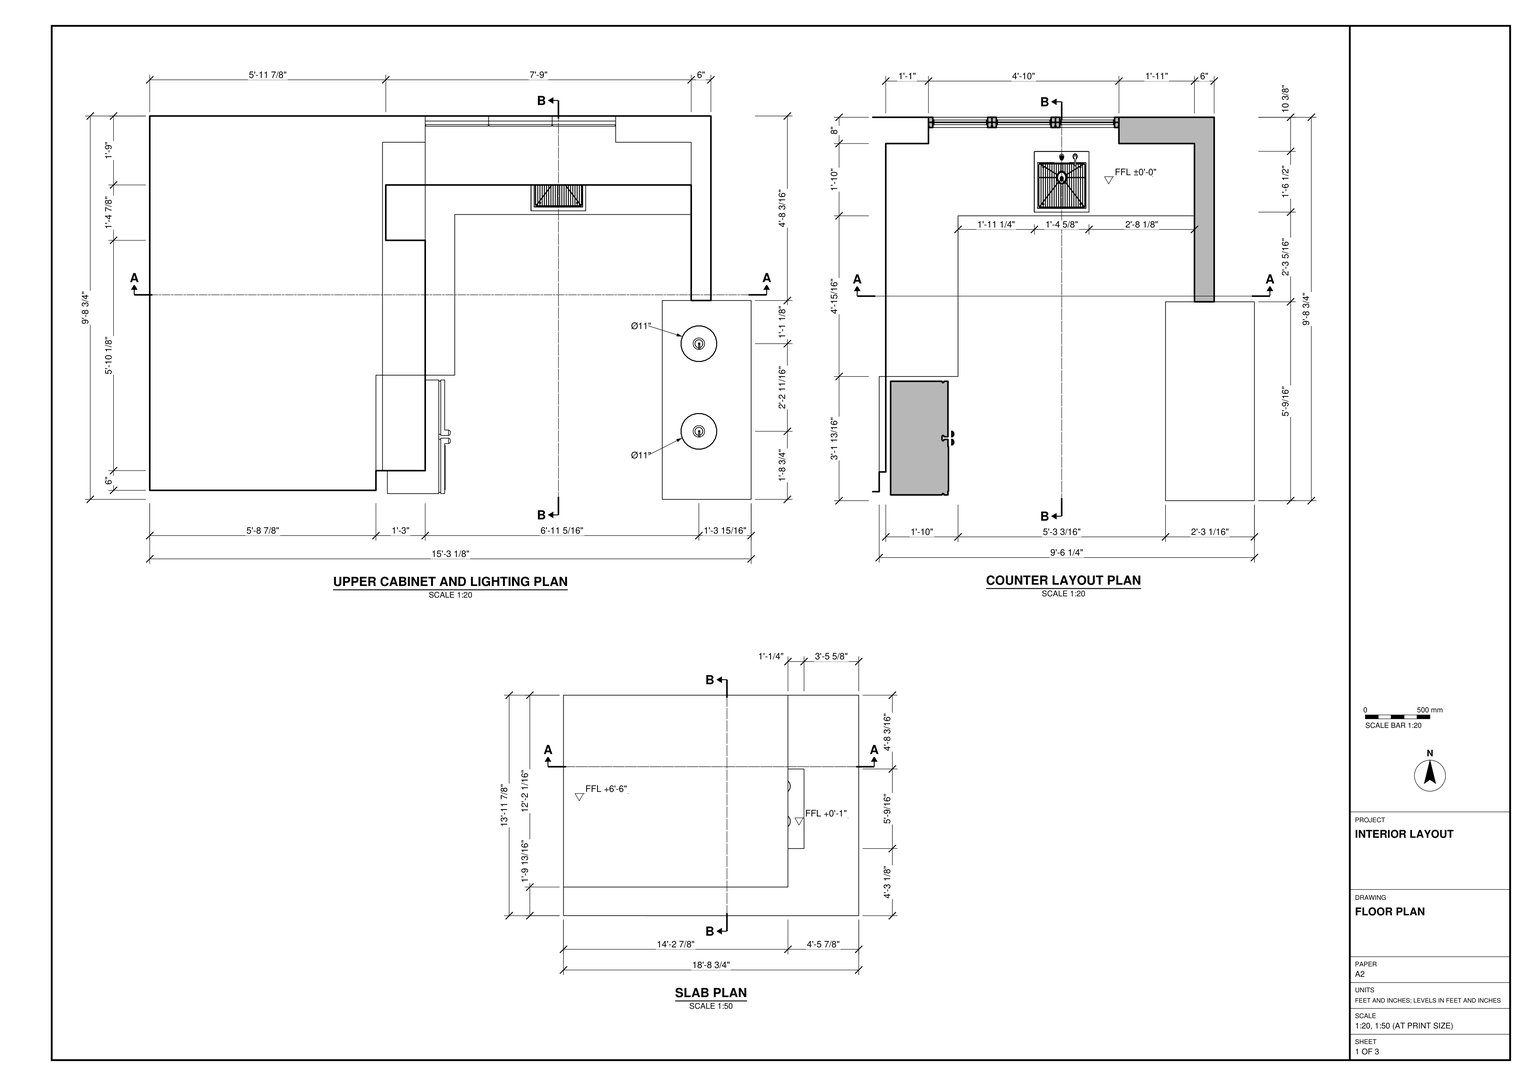
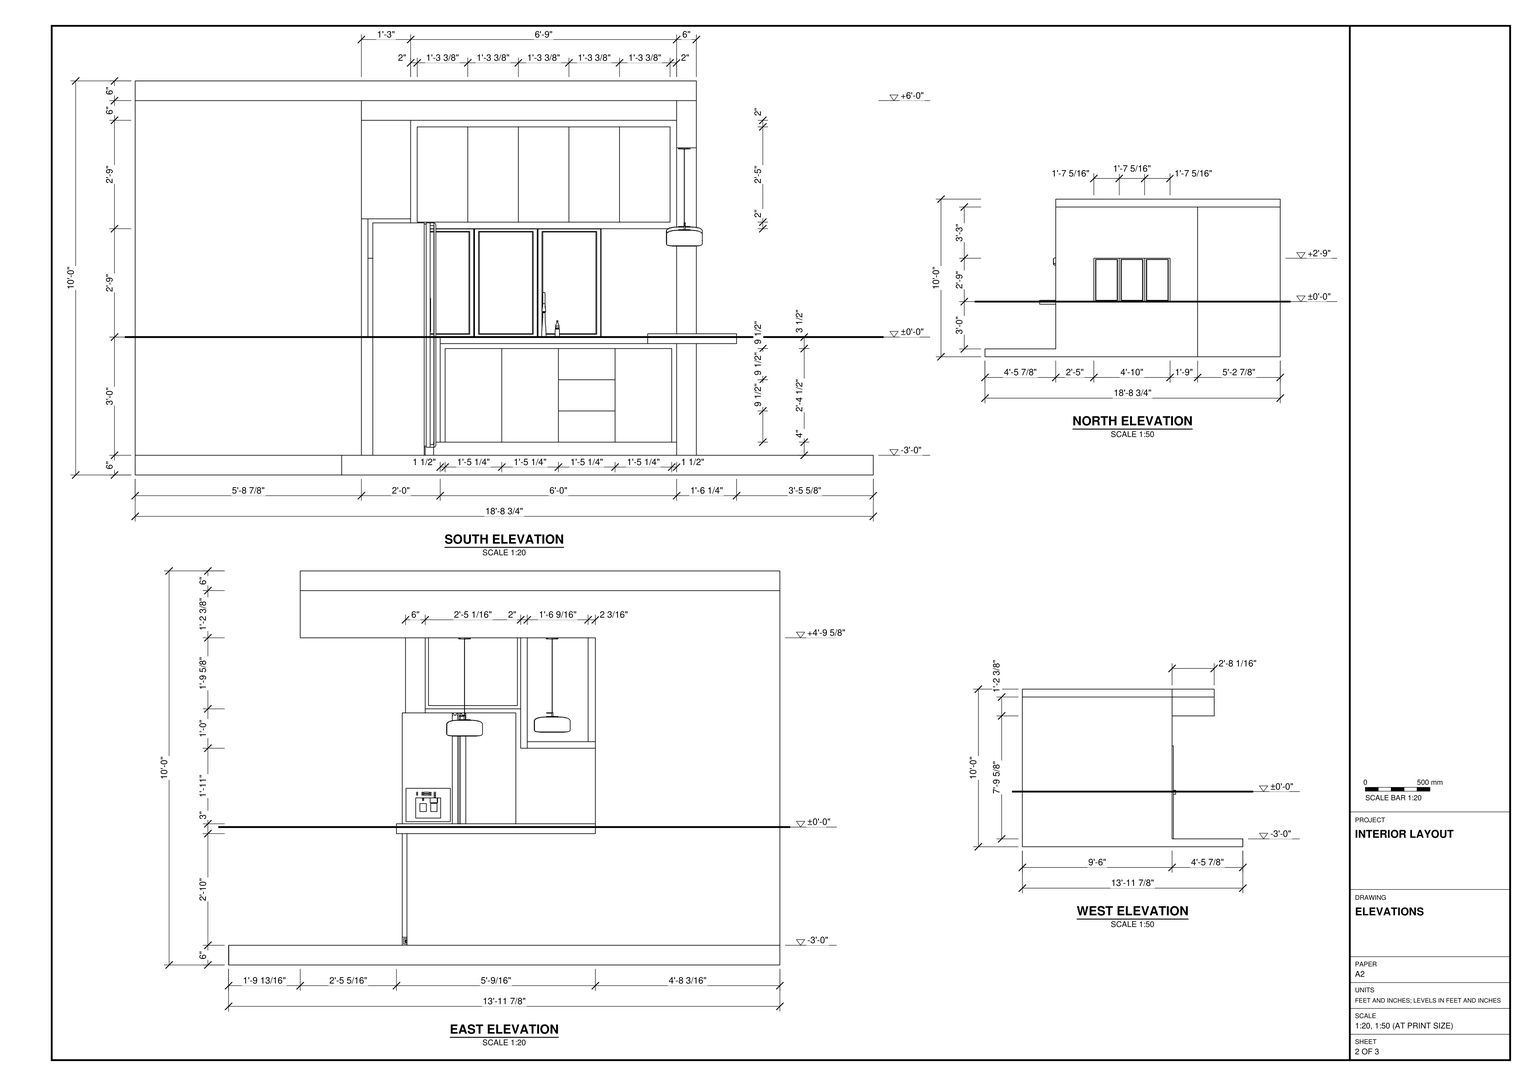
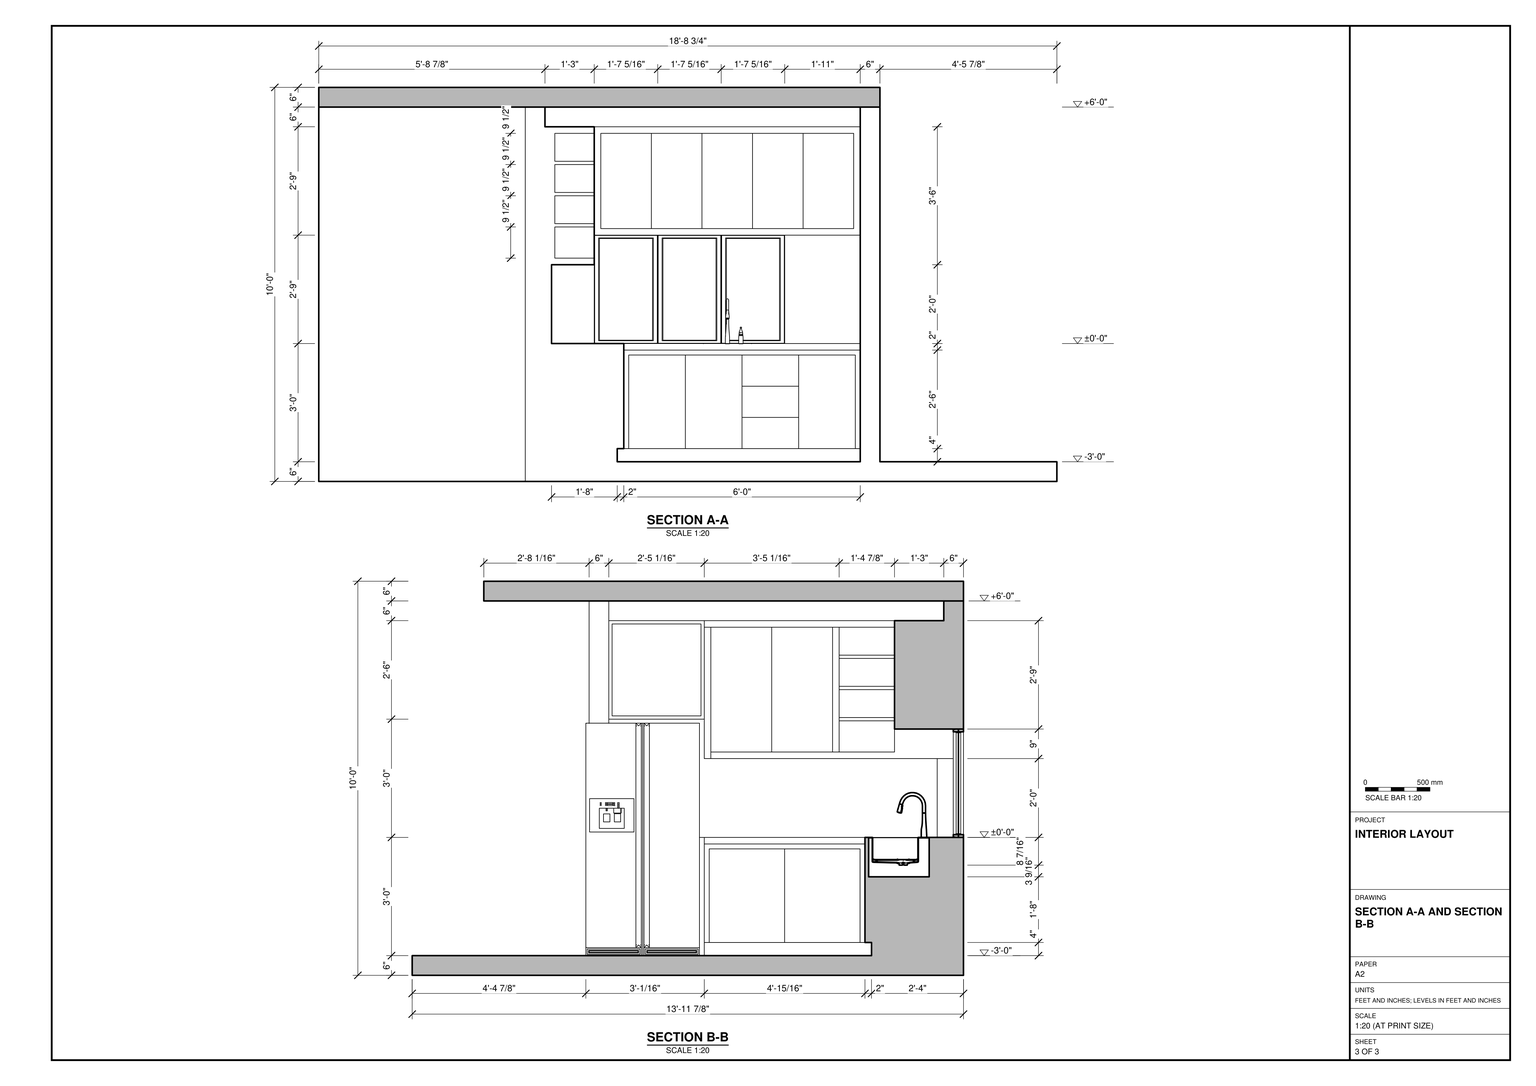
Build the kitchen interior in SketchUp from task_files/diagram_01.pdf. Work in feet and inches. The overall model is 18'-8 3/4" along X, 13'-11 7/8" along Y and 10'-0" high. Use the single reference level ±0'-0" at the sink worktop. The top of the floor slab is at -3'-0" and the underside of the overhead slab is at +6'-0". Use the slab plan for their different footprints and the sections for their thicknesses. Model the walls and returns to the thicknesses drawn, leaving the kitchen open where shown.

Build the L-shaped counter with the sink and faucet below the three-panel window. Follow the elevations for the cupboard fronts, drawer stack and recessed plinth beneath the sink run. Fit the upper cabinets and open shelves around the corner, with space for the tall refrigerator at the end of the return. Place the projecting counter on the opposite side of the aisle and use the lighting plan to position the two lights above it. Appliances, lights, decor and loose items may be any suitable library components.

Keep the walls, floor slab, overhead slab and each furniture or joinery piece in separate groups or components. Use components for repeated parts such as matching cabinet fronts. Save one SketchUp model as output_files/kitchen_with_fitted_cabinets_and_projecting_counter.skp.

# SketchUp Ruby script. Lengths in inches.
U = 1.inch
M = Sketchup.active_model
def pt(a) = Geom::Point3d.new(a.map { |v| v * U })
def face(e, loops, mat)
  f = e.add_face(loops[0].map { |a| pt(a) })
  loops[1..].each { |l| e.add_face(l.map { |a| pt(a) }).erase! }
  f.material = f.back_material = mat if mat
  f
end
# faces: each face lists its corners as indices into pts; further lists are holes
def faces(e, pts, list, mat = nil) = list.each { |f| face(e, (f[0].is_a?(Array) ? f : [f]).map { |l| l.map { |i| pts[i] } }, mat) }
# xy, xz, yz: faces in a plane at the given z, y or x. An outline is a flat list of corners, or four numbers for a rectangle; further outlines are holes
def ring(l) = l.size == 4 ? [[l[0], l[1]], [l[2], l[1]], [l[2], l[3]], [l[0], l[3]]] : l.each_slice(2).to_a
def flat(e, list, mat, &to3) = list.each { |f| face(e, (f[0].is_a?(Array) ? f : [f]).map { |l| ring(l).map { |u, v| to3.(u, v) } }, mat) }
def xy(e, z, list, mat = nil) = flat(e, list, mat) { |x, y| [x, y, z] }
def xz(e, y, list, mat = nil) = flat(e, list, mat) { |x, z| [x, y, z] }
def yz(e, x, list, mat = nil) = flat(e, list, mat) { |y, z| [x, y, z] }
def lines(e, pts, list) = list.each { |a, b| e.add_line(pt(pts[a]), pt(pts[b])) }
# prism: a flat outline (further loops are holes) pulled along v
def prism(e, loops, v, mat = nil)
  f = face(e, loops, mat); d = Geom::Vector3d.new(v.map { |x| x * U })
  f.pushpull(f.normal.samedirection?(d) ? d.length : -d.length)
end
def box(e, o, s, mat = nil) = prism(e, [[o, [o[0] + s[0], o[1], o[2]], [o[0] + s[0], o[1] + s[1], o[2]], [o[0], o[1] + s[1], o[2]]]], [0, 0, s[2]], mat)
def at(x, y, z, deg = 0) = Geom::Transformation.translation(pt([x, y, z])) * Geom::Transformation.rotation(ORIGIN, Z_AXIS, deg.degrees)
def axes(o, x, y, z) = Geom::Transformation.new([*x, 0, *y, 0, *z, 0, *pt(o).to_a, 1])
def part(name) = M.definitions.add(name)
# library, detail: a bought-in or finely detailed component or shape, given as its bounding box
def library(name, o, s) = part(name).tap { |d| box(d.entities, o, s) }
def detail(e, o, s) = box(e.add_group.entities, o, s)
def put(e, d, t, mat = nil) = e.add_instance(d, t).tap { |i| i.material = mat if mat }
def group(e, t, mat = nil) = e.add_group.tap { |g| g.transformation = t; g.material = mat if mat }.entities
root = M.entities
M.materials.add("Wine2").color = [0, 0, 0]
M.materials["Wine2"].alpha = 0
M.materials.add("[0046_Gold]").color = [255, 215, 0]
M.materials.add("[0067_PaleGreen]").color = [152, 251, 152]
M.materials.add("[0070_SpringGreen]").color = [0, 255, 127]
M.materials.add("[0072_DarkSeaGreen]").color = [143, 188, 143]
M.materials.add("[0087_Cyan]").color = [0, 255, 255]
M.materials.add("[0088_Aquamarine]").color = [127, 255, 212]
M.materials.add("[0096_SkyBlue]").color = [135, 206, 235]
M.materials.add("[0117_GhostWhite]").color = [248, 248, 255]
M.materials.add("[0128_White]").color = [255, 255, 255]
M.materials.add("[0130_Gainsboro]").color = [39, 45, 50]
M.materials.add("[0131_Silver]").color = [192, 192, 192]
M.materials.add("[0133_Gray]").color = [128, 128, 128]
M.materials.add("[0134_DimGray]").color = [105, 105, 105]
M.materials.add("[0136_Charcoal]").color = [35, 35, 35]
M.materials.add("[0137_Black]").color = [0, 0, 0]
M.materials.add("[Granite Dark Gray]").color = [69, 68, 68]
c1 = part("Framed glass panel")
xy(c1.entities,0,[[0,-0.98,43.07,0],[0,0,43.07,1.4]],"[0130_Gainsboro]")
xy(c1.entities,0.3,[[0.3,-1.43,42.77,-0.98]],"[0130_Gainsboro]")
xy(c1.entities,2.95,[[2.95,-1.43,40.12,-0.63],[2.95,-0.63,40.12,0],[2.95,0,40.12,0.64],[2.95,0.64,40.12,1.4]],"[0130_Gainsboro]")
xy(c1.entities,3.54,[[3.54,-0.63,39.53,0],[3.54,0,39.53,0.64]],"[0130_Gainsboro]")
xy(c1.entities,111.8125,[[3.54,-0.63,39.53,0],[3.54,0,39.53,0.64]],"[0130_Gainsboro]")
xy(c1.entities,112.4,[[2.95,-1.43,40.12,-0.63],[2.95,-0.63,40.12,0],[2.95,0,40.12,0.64],[2.95,0.64,40.12,1.4]],"[0130_Gainsboro]")
xy(c1.entities,115.05,[[0.3,-1.43,42.77,-0.98]],"[0130_Gainsboro]")
xy(c1.entities,115.35,[[0,-0.98,43.07,0],[0,0,43.07,1.4]],"[0130_Gainsboro]")
xz(c1.entities,-1.43,[[[0.3,0.3,42.77,115.05],[2.95,2.95,40.12,112.4]]],"[0130_Gainsboro]")
xz(c1.entities,-0.98,[[[0,0,43.07,115.35],[0.3,0.3,42.77,115.05]]],"[0130_Gainsboro]")
xz(c1.entities,-0.63,[[[2.95,2.95,40.12,112.4],[3.54,3.54,39.53,111.8125]]],"[0130_Gainsboro]")
xz(c1.entities,0,[[3.54,3.54,39.53,111.8125]],"Wine2")
xz(c1.entities,0,[[[0,0,43.07,115.35],[2.95,2.95,40.12,112.4]],[[2.95,2.95,40.12,112.4],[3.54,3.54,39.53,111.8125]]],"[0130_Gainsboro]")
xz(c1.entities,0.64,[[[2.95,2.95,40.12,112.4],[3.54,3.54,39.53,111.8125]]],"[0130_Gainsboro]")
xz(c1.entities,1.4,[[[0,0,43.07,115.35],[2.95,2.95,40.12,112.4]]],"[0130_Gainsboro]")
yz(c1.entities,0,[[-0.98,0,0,115.35],[0,0,1.4,115.35]],"[0130_Gainsboro]")
yz(c1.entities,0.3,[[-1.43,0.3,-0.98,115.05]],"[0130_Gainsboro]")
yz(c1.entities,2.95,[[-1.43,2.95,-0.63,112.4],[-0.63,2.95,0,112.4],[0,2.95,0.64,112.4],[0.64,2.95,1.4,112.4]],"[0130_Gainsboro]")
yz(c1.entities,3.54,[[-0.63,3.54,0,111.8125],[0,3.54,0.64,111.8125]],"[0130_Gainsboro]")
yz(c1.entities,39.53,[[-0.63,3.54,0,111.8125],[0,3.54,0.64,111.8125]],"[0130_Gainsboro]")
yz(c1.entities,40.12,[[-1.43,2.95,-0.63,112.4],[-0.63,2.95,0,112.4],[0,2.95,0.64,112.4],[0.64,2.95,1.4,112.4]],"[0130_Gainsboro]")
yz(c1.entities,42.77,[[-1.43,0.3,-0.98,115.05]],"[0130_Gainsboro]")
yz(c1.entities,43.07,[[-0.98,0,0,115.35],[0,0,1.4,115.35]],"[0130_Gainsboro]")
c2 = library("3822-1\#1",[-12.47,-11.03,-4.97],[24.94,22.06,9.94])
c3 = library("647\#1",[-5.42,-7.01,-8.07],[10.84,8.15,16.14])
c4 = library("Cubed Ice",[0.01,0,0],[0.63,0.13,0.01])
c5 = library("Crushed Ice",[0.01,0,0],[0.77,0.13,0.01])
c6 = library("Up",[0.01,0,0],[0.17,0.15,0.01])
c7 = library("Down",[0.01,0,0],[0.36,0.12,0.01])
c8 = library("Down\#1",[0.01,0,0],[0.36,0.12,0.01])
c9 = library("Up\#1",[0.01,0,0],[0.17,0.15,0.01])
c10 = library("Temp: 37*",[0.02,0,0],[1.12,0.22,0.01])
c11 = library("Temp: 0*",[0.02,0,0],[0.98,0.22,0.01])
c12 = library("Hold Temperature",[0.01,0,0],[1.21,0.16,0.01])
c13 = library("Deep Freeze",[0.01,0,0],[0.81,0.15,0.01])
c14 = library("Light",[0.01,0,0],[0.32,0.16,0.01])
c15 = library("建立群組\#482",[0,0,0],[10.95,10.95,81.29])
xy(root,0,[[62.875,0,62.875,0.0625,0,0.0625,0,59.875,62.875,59.875,62.875,167.875,224.75,167.875,224.75,0],[0,59.875,62.875,167.875]],"[0128_White]")
xy(root,6,[[[62.875,0,62.875,0.0625,0,0.0625,0,53.875,68.875,53.875,68.875,88.95,90.875,88.95,90.875,139.875,164.875,139.875,164.875,54.3125,170.875,54.3125,170.875,167.875,224.75,167.875,224.75,0],[72.35,52.88,88.31,52.88,88.31,69.77,88,69.77,88,70.59,88.31,70.59,88.31,87.48,72.35,87.48]],[72.35,52.88,72.35,87.48,88.31,87.48,88.31,70.59,88,70.59,88,69.77,88.31,69.77,88.31,52.88]],"[0128_White]")
xy(root,6.41,[[88.01,53.3,88.31,69.36],[88,71.01,88.31,87.07]],"[0137_Black]")
xy(root,6.8125,[[88.01,53.71,88.31,68.95],[88,71.42,88.31,86.66]],"[0137_Black]")
xy(root,7.02,[[88.01,53.91,88.31,68.74],[88,71.625,88.31,86.45]],"[0137_Black]")
xy(root,7.42,[[88.01,53.91,88.31,68.74],[88,71.625,88.31,86.45]],"[0137_Black]")
xy(root,7.62,[[88.01,53.71,88.31,68.95],[88,71.42,88.31,86.66]],"[0137_Black]")
xy(root,8.03,[[88.01,53.3,88.31,69.36],[88,71.01,88.31,87.07]],"[0137_Black]")
xy(root,8.4375,[[88.61,52.88,88.61,69.77,90.95,69.77,90.95,68.12,89.8125,68.12,89.8125,52.88],[88.61,70.59,88.61,87.48,89.8125,87.48,89.8125,72.24,90.95,72.24,90.95,70.59]])
xy(root,8.4375,[[88.01,52.88,88.31,69.77],[88,70.59,88.31,87.48]],"[0137_Black]")
xy(root,9.25,[[89.8125,68.12,91.01,69.77],[89.8125,70.59,91.01,72.24]])
xy(root,10,[[90.875,88.95,92.875,139.875],[92.875,137.875,164.875,139.875]],"[0128_White]")
xy(root,30,[[116.07,138.99,132.75,157.43]],"[0137_Black]")
xy(root,40,[[156.0625,51.125,164.875,111.6875],[164.875,51.125,170.875,54.3125],[170.875,51.125,183.125,111.6875]],"[0137_Black]")
xy(root,42,[[68.875,59.875,70.875,88.95]],"[0128_White]")
xy(root,42,[[[70.875,88.95,92.875,88.95,92.875,137.875,164.875,137.875,164.875,159.875,141.875,159.875,141.875,167.875,83.875,167.875,83.875,159.875,70.875,159.875],[116.07,138.99,132.75,157.43]]],"[0137_Black]")
xy(root,43,[[156.0625,51.125,183.125,111.6875]],"[0137_Black]")
xy(root,43.64,[[89.8125,54.03,89.96,67.54]])
xy(root,44.73,[[88,56.98,89.96,64.58]],"[0136_Charcoal]")
xy(root,46.72,[[88,58.26,88.31,60.22],[88,61.56,88.31,63.48]],"[0134_DimGray]")
xy(root,49.15,[[88,58.26,88.31,60.22]],"[0134_DimGray]")
xy(root,49.21,[[88,61.56,88.31,63.48]],"[0131_Silver]")
xy(root,49.41,[[[88.9375,61.375,88.72,61.43,88.53,61.55,88.36,61.74,88.24,61.99,88.16,62.26,88.14,62.56,88.18,62.85,88.27,63.12,88.41,63.35,88.59,63.52,88.79,63.62,89.01,63.65,89.22,63.6,89.42,63.47,89.59,63.28,89.71,63.04,89.79,62.76,89.8,62.46,89.77,62.17,89.68,61.9,89.54,61.67,89.36,61.5,89.15,61.4],[88.94,61.51,89.13,61.53,89.3125,61.62,89.47,61.77,89.59,61.97,89.67,62.21,89.71,62.47,89.69,62.73,89.625,62.98,89.52,63.19,89.37,63.36,89.19,63.47,89.01,63.52,88.8125,63.49,88.63,63.4,88.48,63.25,88.35,63.05,88.27,62.8125,88.24,62.55,88.26,62.29,88.32,62.05,88.43,61.83,88.58,61.66,88.75,61.55]]])
xy(root,50.09,[[[88.67,59.02,88.64,59.03,88.6,59.05,88.57,59.08,88.54,59.12,88.52,59.22,88.53,59.28,88.54,59.33,88.57,59.37,88.6,59.4,88.64,59.42,88.67,59.43,88.71,59.42,88.75,59.4,88.78,59.37,88.8,59.33,88.82,59.28,88.82,59.17,88.8,59.12,88.78,59.08,88.75,59.05,88.71,59.03],[88.67,59.08,88.73,59.1,88.75,59.125,88.76,59.15,88.77,59.1875,88.78,59.22,88.76,59.3,88.75,59.32,88.73,59.35,88.67,59.37,88.65,59.36,88.62,59.35,88.6,59.32,88.58,59.3,88.57,59.26,88.57,59.1875,88.58,59.15,88.62,59.1,88.65,59.09]]])
xy(root,50.89,[[88.67,59.08,88.65,59.09,88.62,59.1,88.58,59.15,88.57,59.1875,88.57,59.26,88.58,59.3,88.6,59.32,88.62,59.35,88.65,59.36,88.67,59.37,88.73,59.35,88.75,59.32,88.76,59.3,88.78,59.22,88.77,59.1875,88.76,59.15,88.75,59.125,88.73,59.1],[88.94,61.51,88.75,61.55,88.58,61.66,88.43,61.83,88.32,62.05,88.26,62.29,88.24,62.55,88.27,62.8125,88.35,63.05,88.48,63.25,88.63,63.4,88.8125,63.49,89.01,63.52,89.19,63.47,89.37,63.36,89.52,63.19,89.625,62.98,89.69,62.73,89.71,62.47,89.67,62.21,89.59,61.97,89.47,61.77,89.3125,61.62,89.13,61.53]])
xy(root,50.89,[[[88,56.98,89.96,64.58],[88.9375,61.375,89.15,61.4,89.36,61.5,89.54,61.67,89.68,61.9,89.77,62.17,89.8,62.46,89.79,62.76,89.71,63.04,89.59,63.28,89.42,63.47,89.22,63.6,89.01,63.65,88.79,63.62,88.59,63.52,88.41,63.35,88.27,63.12,88.18,62.85,88.14,62.56,88.16,62.26,88.24,61.99,88.36,61.74,88.53,61.55,88.72,61.43],[88.67,59.02,88.71,59.03,88.75,59.05,88.78,59.08,88.8,59.12,88.82,59.17,88.82,59.28,88.8,59.33,88.78,59.37,88.75,59.4,88.71,59.42,88.67,59.43,88.64,59.42,88.6,59.4,88.57,59.37,88.54,59.33,88.53,59.28,88.52,59.22,88.54,59.12,88.57,59.08,88.6,59.05,88.64,59.03]]],"[0136_Charcoal]")
xy(root,53.81,[[89.8125,54.03,89.96,67.54]])
xy(root,66,[[70.875,88.95,83.875,159.875]],"[0128_White]")
xy(root,68,[[71.875,130.01,83.875,146.875]],"[0128_White]")
xy(root,75,[[83.875,146.875,83.875,167.875,141.875,167.875,141.875,159.875,164.875,159.875,164.875,146.875]],"[0128_White]")
xy(root,75.97,[[89.8125,68.12,91.01,69.77],[89.8125,70.59,91.01,72.24]])
xy(root,76.78,[[72.35,52.88,88.01,52.88,88.01,69.77,88,69.77,88,87.48,72.35,87.48],[88.61,52.88,89.8125,52.88,89.8125,68.12,90.95,68.12,90.95,69.77,88.61,69.77],[88.61,70.59,90.95,70.59,90.95,72.24,89.8125,72.24,89.8125,87.48,88.61,87.48]])
xy(root,77.5,[[71.875,130.01,83.875,146.875]],"[0128_White]")
xy(root,78,[[70.875,59.875,83.875,88.95]],"[0128_White]")
xy(root,78.5,[[71.875,130.01,83.875,146.875]],"[0128_White]")
xy(root,87,[[71.875,130.01,83.875,146.875]],"[0128_White]")
xy(root,88,[[71.875,130.01,83.875,146.875]],"[0128_White]")
xy(root,96.5,[[71.875,130.01,83.875,146.875]],"[0128_White]")
xy(root,97.5,[[71.875,130.01,83.875,146.875]],"[0128_White]")
xy(root,99.625,[[164.875,21.8125,170.875,111.6875]],"[0128_White]")
xy(root,106,[[71.875,130.01,83.875,146.875]],"[0128_White]")
xy(root,108,[[68.875,59.875,83.875,59.875,83.875,146.875,164.875,146.875,164.875,161.875,68.875,161.875]],"[0133_Gray]")
xy(root,114,[[0,21.8125,164.875,21.8125,164.875,161.875,68.875,161.875,68.875,53.875,0,53.875],[164.875,21.8125,170.875,21.8125,170.875,167.875,62.875,167.875,62.875,161.875,164.875,161.875],[0,53.875,68.875,53.875,68.875,59.875,62.875,59.875,62.875,167.875,0,167.875],[62.875,59.875,68.875,161.875]],"[0128_White]")
xy(root,120,[[0,21.8125,170.875,167.875]],"[0128_White]")
xz(root,0,[[62.875,0,224.75,6]],"[0128_White]")
xz(root,0.0625,[[0,0,62.875,6]],"[0128_White]")
xz(root,21.8125,[[0,114,170.875,120]])
xz(root,21.8125,[[164.875,99.625,170.875,114]],"[0128_White]")
xz(root,51.125,[[156.0625,40,183.125,43]],"[0137_Black]")
xz(root,52.88,[[72.35,6,88.01,76.78],[88.61,8.4375,89.8125,76.78]])
xz(root,52.88,[[88.01,6,88.31,8.4375]],"[0137_Black]")
xz(root,53.3,[[88.01,6.41,88.31,8.03]],"[0137_Black]")
xz(root,53.71,[[88.01,6.8125,88.31,7.62]],"[0137_Black]")
xz(root,53.875,[[0,6,68.875,114]],"[0128_White]")
xz(root,53.91,[[88.01,7.02,88.31,7.42]],"[0137_Black]")
xz(root,54.03,[[89.8125,43.64,89.96,53.81]])
xz(root,54.3125,[[164.875,6,170.875,40]],"[0128_White]")
xz(root,56.98,[[88,44.73,89.96,50.89]],"[0136_Charcoal]")
xz(root,58.26,[[88,46.72,88.31,49.15]],"[0134_DimGray]")
xz(root,59.875,[[68.875,42,70.875,78]],"[0128_White]")
xz(root,59.875,[[68.875,78,83.875,108]],"[0133_Gray]")
xz(root,60.22,[[88,46.72,88.31,49.15]],"[0134_DimGray]")
xz(root,61.56,[[88,46.72,88.31,49.21]],"[0134_DimGray]")
xz(root,63.48,[[88,46.72,88.31,49.21]],"[0134_DimGray]")
xz(root,64.58,[[88,44.73,89.96,50.89]],"[0136_Charcoal]")
xz(root,67.54,[[89.8125,43.64,89.96,53.81]])
xz(root,68.12,[[89.8125,8.4375,90.95,9.25],[89.8125,75.97,90.95,76.78]])
xz(root,68.74,[[88.01,7.02,88.31,7.42]],"[0137_Black]")
xz(root,68.95,[[88.01,6.8125,88.31,7.62]],"[0137_Black]")
xz(root,69.36,[[88.01,6.41,88.31,8.03]],"[0137_Black]")
xz(root,69.77,[[88.61,8.4375,88.61,76.78,90.95,76.78,90.95,75.97,89.8125,75.97,89.8125,9.25,90.95,9.25,90.95,8.4375]])
xz(root,69.77,[[88,6,88,76.78,88.01,76.78,88.01,8.4375,88.31,8.4375,88.31,6]],"[0137_Black]")
xz(root,70.59,[[88.61,8.4375,90.95,8.4375,90.95,9.25,89.8125,9.25,89.8125,75.97,90.95,75.97,90.95,76.78,88.61,76.78]])
xz(root,70.59,[[88,6,88.31,8.4375]],"[0137_Black]")
xz(root,71.01,[[88,6.41,88.31,8.03]],"[0137_Black]")
xz(root,71.42,[[88,6.8125,88.31,7.62]],"[0137_Black]")
xz(root,71.625,[[88,7.02,88.31,7.42]],"[0137_Black]")
xz(root,72.24,[[89.8125,8.4375,90.95,9.25],[89.8125,75.97,90.95,76.78]])
xz(root,86.45,[[88,7.02,88.31,7.42]],"[0137_Black]")
xz(root,86.66,[[88,6.8125,88.31,7.62]],"[0137_Black]")
xz(root,87.07,[[88,6.41,88.31,8.03]],"[0137_Black]")
xz(root,87.48,[[72.35,6,88,76.78],[88.61,8.4375,89.8125,76.78]])
xz(root,87.48,[[88,6,88.31,8.4375]],"[0137_Black]")
xz(root,88.95,[[70.875,66,83.875,78]],"[0133_Gray]")
xz(root,88.95,[[68.875,6,90.875,6,90.875,10,92.875,10,92.875,42,68.875,42]],"[0137_Black]")
xz(root,111.6875,[[164.875,43,170.875,99.625]],"[0128_White]")
xz(root,111.6875,[[170.875,40,183.125,43]],"[0137_Black]")
xz(root,111.6875,[[156.0625,40,164.875,42],[156.0625,42,164.875,43]],"[Granite Dark Gray]")
xz(root,130.01,[[71.875,68,83.875,77.5],[71.875,78.5,83.875,87],[71.875,88,83.875,96.5],[71.875,97.5,83.875,106]],"[0128_White]")
xz(root,137.875,[[92.875,10,94.375,10,94.375,38.5,163.375,38.5,163.375,10,164.875,10,164.875,40,92.875,40],[94.375,10,111.625,38.5],[111.625,10,128.875,38.5],[128.875,10,146.125,19.5],[146.125,10,163.375,38.5],
  [128.875,19.5,146.125,29],[128.875,29,146.125,38.5]],"[0133_Gray]")
xz(root,137.875,[[92.875,40,164.875,42]],"[0137_Black]")
xz(root,138.99,[[116.07,30,132.75,42]],"[0137_Black]")
xz(root,139.875,[[90.875,6,164.875,10]],"[0133_Gray]")
xz(root,146.875,[[71.875,68,83.875,75],[[71.875,75,164.875,75,164.875,108,83.875,108,83.875,106,71.875,106,71.875,97.5,83.875,97.5,83.875,96.5,71.875,96.5,71.875,88,83.875,88,83.875,87,71.875,87,71.875,78.5,83.875,78.5,83.875,77.5,71.875,77.5],[85.875,77,162.875,106]],[85.875,77,101.28,106],[101.28,77,116.68,106],[116.68,77,132.07,106],
  [132.07,77,147.48,106],[147.48,77,162.875,106]],"[0133_Gray]")
xz(root,157.43,[[116.07,30,132.75,42]],"[0137_Black]")
xz(root,159.875,[[70.875,42,83.875,66],[141.875,42,164.875,75]],"[0133_Gray]")
xz(root,161.875,[[68.875,108,164.875,114]],"[0128_White]")
xz(root,167.875,[[0,114,170.875,120]])
xz(root,167.875,[[0,0,62.875,114],[[62.875,0,62.875,114,170.875,114,170.875,6,224.75,6,224.75,0],[83.875,42,141.875,75]]],"[0128_White]")
yz(root,0,[[21.8125,114,53.875,120],[53.875,114,167.875,120]])
yz(root,0,[[0.0625,0,0.0625,6,53.875,6,53.875,114,167.875,114,167.875,0]],"[0128_White]")
yz(root,62.875,[[0,0,0.0625,6]],"[0128_White]")
yz(root,68.875,[[53.875,6,88.95,6,88.95,42,59.875,42,59.875,114,53.875,114],[59.875,108,161.875,114]],"[0128_White]")
yz(root,70.875,[[59.875,42,159.875,42,159.875,66,88.95,66,88.95,78,59.875,78]],"[0128_White]")
yz(root,71.875,[[130.01,68,146.875,77.5],[130.01,78.5,146.875,87],[130.01,88,146.875,96.5],[130.01,97.5,146.875,106]],"[0133_Gray]")
yz(root,72.35,[[52.88,6,87.48,76.78]])
yz(root,83.875,[[159.875,42,167.875,66],[88.95,66,90.95,106],[90.95,66,167.875,66,167.875,75,146.875,75,146.875,68,90.95,68],[90.95,68,109.48,106],[109.48,68,128.01,106],
  [128.01,68,130.01,106],[130.01,77.5,146.875,78.5],[[59.875,78,88.95,108],[60.875,79,87.95,107]],[60.875,79,87.95,107],[130.01,87,146.875,88],
  [130.01,96.5,146.875,97.5],[88.95,106,146.875,108]],"[0133_Gray]")
yz(root,88,[[69.77,6,70.18,76.78],[70.18,6,70.59,76.78]])
yz(root,88,[[[71.01,6.41,87.07,8.03],[71.42,6.8125,86.66,7.62]],[71.625,7.02,86.45,7.42]],"[0134_DimGray]")
yz(root,88,[[[56.98,44.73,64.58,50.89],[61.56,46.72,63.48,49.21],[58.26,46.72,60.22,49.15]]],"[0136_Charcoal]")
yz(root,88.01,[[[53.3,6.41,69.36,8.03],[53.71,6.8125,68.95,7.62]],[53.91,7.02,68.74,7.42]],"[0134_DimGray]")
yz(root,88.31,[[58.26,46.72,60.22,49.15],[61.56,46.72,63.48,49.21]],"[0134_DimGray]")
yz(root,88.31,[[[52.88,6,69.77,8.4375],[53.3,6.41,69.36,8.03]],[[70.59,6,87.48,8.4375],[71.01,6.41,87.07,8.03]],[[53.71,6.8125,68.95,7.62],[53.91,7.02,68.74,7.42]],[[71.42,6.8125,86.66,7.62],[71.625,7.02,86.45,7.42]]],"[0137_Black]")
yz(root,88.57,[[59.1875,50.09,59.22,50.89],[59.22,50.09,59.26,50.89]])
yz(root,88.82,[[59.17,50.09,59.22,50.89],[59.22,50.09,59.28,50.89]])
yz(root,89.8125,[[[52.88,8.4375,68.12,8.4375,68.12,9.25,69.77,9.25,69.77,75.97,68.12,75.97,68.12,76.78,52.88,76.78],[54.03,43.64,67.54,53.81]],[72.24,8.4375,87.48,8.4375,87.48,76.78,72.24,76.78,72.24,75.97,70.59,75.97,70.59,9.25,72.24,9.25]])
yz(root,89.96,[[61.47,51.63,61.52,51.63,61.57,51.64,61.62,51.66,61.66,51.7,61.69,51.74,61.71,51.79,61.71,51.85,61.7,51.9,61.68,51.94,61.64,51.98,61.6,52.01,61.54,52.03,61.49,52.03,61.4375,52.02,61.39,52,61.35,51.96,61.32,51.92,61.3,51.87,61.3,51.81,61.3125,51.76,61.34,51.72,61.37,51.68,61.42,51.65],[59.02,51.68,59.08,51.69,59.125,51.71,59.17,51.74,59.2,51.79,59.22,51.83,59.23,51.89,59.22,51.94,59.2,51.99,59.17,52.03,59.125,52.0625,59.08,52.08,59.02,52.09,58.97,52.08,58.92,52.0625,58.88,52.03,58.85,51.99,58.82,51.94,58.82,51.83,58.85,51.79,58.88,51.74,58.92,51.71,58.97,51.69],[61.5,52.22,61.55,52.23,61.6,52.25,61.64,52.28,61.68,52.32,61.7,52.37,61.7,52.48,61.68,52.53,61.64,52.57,61.6,52.6,61.55,52.62,61.5,52.63,61.44,52.62,61.39,52.6,61.35,52.57,61.32,52.53,61.3,52.48,61.29,52.42,61.3,52.37,61.32,52.32,61.35,52.28,61.39,52.25,61.44,52.23],[58.97,52.24,59.08,52.24,59.17,52.3,59.2,52.34,59.22,52.39,59.23,52.44,59.22,52.49,59.2,52.54,59.17,52.59,59.125,52.62,59.08,52.64,58.97,52.64,58.92,52.62,58.88,52.59,58.82,52.49,58.82,52.39,58.85,52.34,58.88,52.3,58.92,52.27]],"[0046_Gold]")
yz(root,89.96,[[62.57,52.17,63.03,52.62]],"[0067_PaleGreen]")
yz(root,89.96,[[62.57,51.61,63.03,52.0625]],"[0070_SpringGreen]")
yz(root,89.96,[[62.57,51.05,63.03,51.5]],"[0072_DarkSeaGreen]")
yz(root,89.96,[[57.41,51.68,57.46,51.69,57.51,51.71,57.55,51.74,57.59,51.79,57.61,51.83,57.61,51.94,57.59,51.99,57.55,52.03,57.51,52.0625,57.46,52.08,57.41,52.09,57.35,52.08,57.31,52.0625,57.26,52.03,57.23,51.99,57.21,51.94,57.2,51.89,57.21,51.83,57.23,51.79,57.26,51.74,57.31,51.71,57.35,51.69]],"[0087_Cyan]")
yz(root,89.96,[[57.41,52.24,57.46,52.24,57.51,52.26,57.55,52.3,57.58,52.34,57.61,52.39,57.61,52.49,57.59,52.54,57.56,52.58,57.51,52.62,57.46,52.64,57.36,52.64,57.31,52.62,57.26,52.59,57.23,52.55,57.21,52.5,57.2,52.44,57.21,52.39,57.23,52.34,57.26,52.3,57.3,52.27,57.35,52.25]],"[0088_Aquamarine]")
yz(root,89.96,[[59.43,51.68,61.08,52.08],[59.45,52.23,61.1,52.62]],"[0096_SkyBlue]")
yz(root,89.96,[[[54.03,43.64,67.54,53.81],[56.98,44.73,64.58,50.89],[59.45,52.23,61.1,52.62],[59.43,51.68,61.08,52.08],[62.57,52.17,63.03,52.62],[62.57,51.05,63.03,51.5],[62.57,51.61,63.03,52.0625],[57.41,52.24,57.35,52.25,57.3,52.27,57.26,52.3,57.23,52.34,57.21,52.39,57.2,52.44,57.21,52.5,57.23,52.55,57.26,52.59,57.31,52.62,57.36,52.64,57.46,52.64,57.51,52.62,57.56,52.58,57.59,52.54,57.61,52.49,57.61,52.39,57.58,52.34,57.55,52.3,57.51,52.26,57.46,52.24],[61.5,52.22,61.44,52.23,61.39,52.25,61.35,52.28,61.32,52.32,61.3,52.37,61.29,52.42,61.3,52.48,61.32,52.53,61.35,52.57,61.39,52.6,61.44,52.62,61.5,52.63,61.55,52.62,61.6,52.6,61.64,52.57,61.68,52.53,61.7,52.48,61.7,52.37,61.68,52.32,61.64,52.28,61.6,52.25,61.55,52.23],[57.41,51.68,57.35,51.69,57.31,51.71,57.26,51.74,57.23,51.79,57.21,51.83,57.2,51.89,57.21,51.94,57.23,51.99,57.26,52.03,57.31,52.0625,57.35,52.08,57.41,52.09,57.46,52.08,57.51,52.0625,57.55,52.03,57.59,51.99,57.61,51.94,57.61,51.83,57.59,51.79,57.55,51.74,57.51,51.71,57.46,51.69],[59.02,51.68,58.97,51.69,58.92,51.71,58.88,51.74,58.85,51.79,58.82,51.83,58.82,51.94,58.85,51.99,58.88,52.03,58.92,52.0625,58.97,52.08,59.02,52.09,59.08,52.08,59.125,52.0625,59.17,52.03,59.2,51.99,59.22,51.94,59.23,51.89,59.22,51.83,59.2,51.79,59.17,51.74,59.125,51.71,59.08,51.69],[58.97,52.24,58.92,52.27,58.88,52.3,58.85,52.34,58.82,52.39,58.82,52.49,58.88,52.59,58.92,52.62,58.97,52.64,59.08,52.64,59.125,52.62,59.17,52.59,59.2,52.54,59.22,52.49,59.23,52.44,59.22,52.39,59.2,52.34,59.17,52.3,59.08,52.24],[61.47,51.63,61.42,51.65,61.37,51.68,61.34,51.72,61.3125,51.76,61.3,51.81,61.3,51.87,61.32,51.92,61.35,51.96,61.39,52,61.4375,52.02,61.49,52.03,61.54,52.03,61.6,52.01,61.64,51.98,61.68,51.94,61.7,51.9,61.71,51.85,61.71,51.79,61.69,51.74,61.66,51.7,61.62,51.66,61.57,51.64,61.52,51.63]]],"[0136_Charcoal]")
yz(root,90.875,[[88.95,6,139.875,10]],"[0133_Gray]")
yz(root,91.01,[[68.12,9.25,69.77,75.97],[70.59,9.25,72.24,75.97]])
yz(root,92.875,[[88.95,10,90.45,10,90.45,38.5,136.375,38.5,136.375,10,137.875,10,137.875,40,88.95,40],[90.45,10,113.41,38.5],[113.41,10,136.375,38.5]],"[0133_Gray]")
yz(root,92.875,[[88.95,40,137.875,42]],"[0137_Black]")
yz(root,116.07,[[138.99,30,157.43,42]],"[0137_Black]")
yz(root,132.75,[[138.99,30,157.43,42]],"[0137_Black]")
yz(root,141.875,[[159.875,42,167.875,75]],"[0133_Gray]")
yz(root,156.0625,[[51.125,40,111.6875,43]],"[0137_Black]")
yz(root,164.875,[[54.3125,6,54.3125,40,111.6875,40,111.6875,108,146.875,108,146.875,75,159.875,75,159.875,42,137.875,42,137.875,10,139.875,10,139.875,6],[137.875,10,139.875,40],[21.8125,99.625,21.8125,114,161.875,114,161.875,108,111.6875,108,111.6875,99.625]],"[0128_White]")
yz(root,170.875,[[21.8125,114,167.875,120]])
yz(root,170.875,[[54.3125,6,167.875,6,167.875,114,21.8125,114,21.8125,99.625,111.6875,99.625,111.6875,40,54.3125,40]],"[0128_White]")
yz(root,183.125,[[51.125,40,111.6875,43]],"[0137_Black]")
yz(root,224.75,[[0,0,167.875,6]],"[0128_White]")
p = [[88.01,69.77,8.4375],[88.02,69.66,8.54],[88.02,52.99,8.54],[88.01,52.88,8.4375],[88.02,52.99,76.68],[88.01,52.88,76.78],
  [88.6,69.66,8.54],[88.61,69.77,8.4375],[88.61,52.88,8.4375],[88.6,52.99,8.54],[88.61,52.88,76.78],[88.6,52.99,76.68],
  [91.11,68.15,8.46],[90.95,68.12,8.4375],[90.95,69.77,8.4375],[91.11,69.74,8.46],[91.11,68.15,76.75],[90.95,68.12,76.78],
  [90.95,68.12,75.97],[90.95,68.12,75.15],[90.95,68.12,10.0625],[90.95,68.12,9.25],[91.11,68.15,10.04],[91.11,68.15,75.18],
  [88.01,69.77,76.78],[88.02,69.66,76.68],[88.6,69.66,76.68],[88.61,69.77,76.78],[90.95,69.77,9.25],[90.95,69.77,10.0625],
  [90.95,69.77,75.15],[90.95,69.77,75.97],[90.95,69.77,76.78],[91.11,69.74,76.75],[91.11,69.74,75.18],[91.11,69.74,10.04],
  [88,87.48,8.4375],[88.02,87.37,8.54],[88.02,70.7,8.54],[88,70.59,8.4375],[88.02,70.7,76.68],[88,70.59,76.78],
  [88.6,87.37,8.54],[88.61,87.48,8.4375],[88.61,70.59,8.4375],[88.6,70.7,8.54],[88.61,70.59,76.78],[88.6,70.7,76.68],
  [90.95,72.24,8.4375],[91.11,72.21,8.46],[91.11,70.62,8.46],[90.95,70.59,8.4375],[91.11,70.62,10.04],[91.11,70.62,75.18],
  [91.11,70.62,76.75],[90.95,70.59,76.78],[90.95,70.59,75.97],[90.95,70.59,75.15],[90.95,70.59,10.0625],[90.95,70.59,9.25],
  [90.95,72.24,76.78],[91.11,72.21,76.75],[91.11,72.21,75.18],[91.11,72.21,10.04],[90.95,72.24,9.25],[90.95,72.24,10.0625],
  [90.95,72.24,75.15],[90.95,72.24,75.97],[88,87.48,76.78],[88.02,87.37,76.68],[88.6,87.37,76.68],[88.61,87.48,76.78],
  [88.05,69.5625,8.64],[88.05,53.09,8.64],[88.05,53.09,76.58],[88.57,69.5625,8.64],[88.57,53.09,8.64],[88.57,53.09,76.58],
  [91.25,68.23,8.55],[91.25,69.66,8.55],[91.25,68.23,76.67],[91.25,68.23,9.95],[91.25,68.23,75.26],[91.38,68.36,8.67],
  [91.38,69.53,8.67],[91.38,68.36,76.54],[91.38,68.36,9.82],[91.38,68.36,75.39],[91.25,69.66,9.95],[91.25,69.66,75.26],
  [91.25,69.66,76.67],[91.38,69.53,76.54],[91.38,69.53,75.39],[91.38,69.53,9.82],[88.05,69.5625,76.58],[88.57,69.5625,76.58],
  [91.25,72.13,8.55],[91.25,70.7,8.55],[91.25,70.7,9.95],[91.25,70.7,75.26],[91.25,70.7,76.67],[88.05,87.27,8.64],
  [88.05,70.8,8.64],[88.05,70.8,76.58],[88.57,87.27,8.64],[88.57,70.8,8.64],[88.57,70.8,76.58],[91.38,72,8.67],
  [91.38,70.84,8.67],[91.38,70.84,9.82],[91.38,70.84,75.39],[91.38,70.84,76.54],[91.25,72.13,76.67],[91.38,72,76.54],
  [91.38,72,75.39],[91.38,72,9.82],[91.25,72.13,9.95],[91.25,72.13,75.26],[88.05,87.27,76.58],[88.57,87.27,76.58],
  [88.09,69.48,8.72],[88.09,53.18,8.72],[88.09,53.18,76.49],[88.52,69.48,8.72],[88.52,53.18,8.72],[88.52,53.18,76.49],
  [88.09,69.48,76.49],[88.52,69.48,76.49],[88.09,87.1875,8.72],[88.09,70.89,8.72],[88.09,70.89,76.49],[88.52,87.1875,8.72],
  [88.52,70.89,8.72],[88.52,70.89,76.49],[88.09,87.1875,76.49],[88.52,87.1875,76.49],[88.16,69.41,8.79],[88.16,53.24,8.79],
  [88.16,53.24,76.43],[88.46,69.41,8.79],[88.46,53.24,8.79],[88.46,53.24,76.43],[91.48,68.53,8.84],[91.48,69.36,8.84],
  [91.48,68.53,76.375],[91.48,68.53,9.66],[91.48,68.53,75.56],[88.16,69.41,76.43],[88.46,69.41,76.43],[91.48,69.36,76.375],
  [91.48,69.36,75.56],[91.48,69.36,9.66],[91.48,71.83,8.84],[91.48,71.01,8.84],[91.48,71.01,9.66],[91.48,71.01,75.56],
  [91.48,71.01,76.375],[88.16,87.12,8.79],[88.16,70.95,8.79],[88.16,70.95,76.43],[88.46,87.12,8.79],[88.46,70.95,8.79],
  [88.46,70.95,76.43],[91.48,71.83,76.375],[91.48,71.83,75.56],[91.48,71.83,9.66],[88.16,87.12,76.43],[88.46,87.12,76.43],
  [88.23,69.37,8.83],[88.23,53.28,8.83],[88.23,53.28,76.39],[88.39,69.37,8.83],[88.39,53.28,8.83],[88.39,53.28,76.39],
  [88.31,69.36,8.84],[88.31,53.3,8.84],[88.31,53.3,76.37],[91.54,68.73,9.04],[91.54,69.16,9.04],[91.54,68.73,76.18],
  [91.54,68.73,9.46],[91.54,68.73,75.76],[91.54,69.16,76.18],[91.54,69.16,75.76],[91.54,69.16,9.46],[88.23,69.37,76.39],
  [88.31,69.36,76.37],[88.39,69.37,76.39],[88.23,87.08,8.83],[88.31,87.07,8.84],[88.31,71.01,8.84],[88.23,70.99,8.83],
  [88.31,71.01,76.375],[88.23,70.99,76.39],[88.38,87.08,8.83],[88.38,70.99,8.83],[88.38,70.99,76.39],[91.54,71.63,9.04],
  [91.54,71.2,9.04],[91.54,71.2,9.46],[91.54,71.2,75.76],[91.54,71.2,76.18],[91.54,71.63,76.18],[91.54,71.63,75.76],
  [91.54,71.63,9.46],[88.23,87.08,76.39],[88.31,87.07,76.375],[88.38,87.08,76.39],[91.56,68.95,9.25],[91.56,68.95,75.97],
  [91.56,71.42,9.25],[91.56,71.42,75.97],[88.72,61.43,50.89],[88.53,61.55,50.89],[88.53,61.55,49.41],[88.72,61.43,49.41],
  [88.9375,61.375,50.89],[88.9375,61.375,49.41],[89.15,61.4,50.89],[89.15,61.4,49.41],[89.36,61.5,50.89],[89.36,61.5,49.41],
  [88.75,61.55,50.89],[88.94,61.51,50.89],[88.94,61.51,49.41],[88.75,61.55,49.41],[89.13,61.53,50.89],[89.13,61.53,49.41],
  [89.3125,61.62,50.89],[89.3125,61.62,49.41],[89.54,61.67,50.89],[89.54,61.67,49.41],[88.36,61.74,50.89],[88.36,61.74,49.41],
  [88.58,61.66,50.89],[88.58,61.66,49.41],[89.47,61.77,50.89],[89.47,61.77,49.41],[88.24,61.99,50.89],[88.24,61.99,49.41],
  [88.43,61.83,50.89],[88.43,61.83,49.41],[89.68,61.9,50.89],[89.68,61.9,49.41],[88.32,62.05,50.89],[88.32,62.05,49.41],
  [89.59,61.97,50.89],[89.59,61.97,49.41],[89.77,62.17,50.89],[89.77,62.17,49.41],[88.16,62.26,50.89],[88.16,62.26,49.41],
  [88.26,62.29,50.89],[88.26,62.29,49.41],[89.67,62.21,50.89],[89.67,62.21,49.41],[89.71,62.47,50.89],[89.71,62.47,49.41],
  [89.8,62.46,50.89],[89.8,62.46,49.41],[88.14,62.56,50.89],[88.14,62.56,49.41],[88.24,62.55,50.89],[88.24,62.55,49.41],
  [89.69,62.73,50.89],[89.69,62.73,49.41],[89.79,62.76,50.89],[89.79,62.76,49.41],[88.18,62.85,50.89],[88.18,62.85,49.41],
  [88.27,62.8125,50.89],[88.27,62.8125,49.41],[89.625,62.98,50.89],[89.625,62.98,49.41],[88.35,63.05,50.89],[88.35,63.05,49.41],
  [89.71,63.04,50.89],[89.71,63.04,49.41],[88.27,63.12,50.89],[88.27,63.12,49.41],[89.52,63.19,50.89],[89.52,63.19,49.41],
  [89.59,63.28,50.89],[89.59,63.28,49.41],[88.41,63.35,50.89],[88.41,63.35,49.41],[88.48,63.25,50.89],[88.48,63.25,49.41],
  [89.37,63.36,50.89],[89.37,63.36,49.41],[88.63,63.4,50.89],[88.63,63.4,49.41],[89.42,63.47,50.89],[89.42,63.47,49.41],
  [88.59,63.52,50.89],[88.59,63.52,49.41],[88.8125,63.49,50.89],[88.8125,63.49,49.41],[89.19,63.47,50.89],[89.19,63.47,49.41],
  [88.79,63.62,50.89],[88.79,63.62,49.41],[89.01,63.52,50.89],[89.01,63.52,49.41],[89.22,63.6,50.89],[89.22,63.6,49.41],
  [89.01,63.65,50.89],[89.01,63.65,49.41],[88.67,59.02,50.89],[88.64,59.03,50.89],[88.64,59.03,50.09],[88.67,59.02,50.09],
  [88.6,59.05,50.89],[88.6,59.05,50.09],[88.57,59.08,50.89],[88.57,59.08,50.09],[88.78,59.08,50.89],[88.75,59.05,50.89],
  [88.75,59.05,50.09],[88.78,59.08,50.09],[88.71,59.03,50.89],[88.71,59.03,50.09],[88.54,59.12,50.89],[88.54,59.12,50.09],
  [88.53,59.17,50.89],[88.53,59.17,50.09],[88.58,59.15,50.89],[88.6,59.125,50.89],[88.6,59.125,50.09],[88.58,59.15,50.09],
  [88.62,59.1,50.89],[88.62,59.1,50.09],[88.65,59.09,50.89],[88.65,59.09,50.09],[88.67,59.08,50.89],[88.67,59.08,50.09],
  [88.7,59.09,50.89],[88.7,59.09,50.09],[88.73,59.1,50.89],[88.73,59.1,50.09],[88.75,59.125,50.89],[88.75,59.125,50.09],
  [88.76,59.15,50.89],[88.76,59.15,50.09],[88.82,59.17,50.89],[88.8,59.12,50.89],[88.8,59.12,50.09],[88.82,59.17,50.09],
  [88.52,59.22,50.89],[88.52,59.22,50.09],[88.53,59.28,50.89],[88.53,59.28,50.09],[88.57,59.1875,50.89],[88.57,59.1875,50.09],
  [88.77,59.1875,50.89],[88.78,59.22,50.89],[88.78,59.22,50.09],[88.77,59.1875,50.09],[88.77,59.26,50.89],[88.77,59.26,50.09],
  [88.54,59.33,50.89],[88.54,59.33,50.09],[88.57,59.37,50.89],[88.57,59.37,50.09],[88.65,59.36,50.89],[88.62,59.35,50.89],
  [88.62,59.35,50.09],[88.65,59.36,50.09],[88.6,59.32,50.89],[88.6,59.32,50.09],[88.58,59.3,50.89],[88.58,59.3,50.09],
  [88.57,59.26,50.89],[88.57,59.26,50.09],[88.76,59.3,50.89],[88.75,59.32,50.89],[88.75,59.32,50.09],[88.76,59.3,50.09],
  [88.73,59.35,50.89],[88.73,59.35,50.09],[88.7,59.36,50.89],[88.7,59.36,50.09],[88.78,59.37,50.89],[88.8,59.33,50.89],
  [88.8,59.33,50.09],[88.78,59.37,50.09],[88.82,59.28,50.89],[88.82,59.28,50.09],[88.6,59.4,50.89],[88.6,59.4,50.09],
  [88.64,59.42,50.89],[88.64,59.42,50.09],[88.67,59.43,50.89],[88.67,59.43,50.09],[88.67,59.37,50.89],[88.67,59.37,50.09],
  [88.71,59.42,50.89],[88.71,59.42,50.09],[88.75,59.4,50.89],[88.75,59.4,50.09]]
faces(root,p,[[0,1,2,3],[3,2,4,5],[6,7,8,9],[9,8,10,11],[24,25,1,0],[26,27,7,6],[36,37,38,39],[39,38,40,41],
  [42,43,44,45],[45,44,46,47],[68,69,37,36],[70,71,43,42],[1,72,73,2],[2,73,74,4],[75,6,9,76],[76,9,11,77],
  [25,94,72,1],[95,26,6,75],[37,101,102,38],[38,102,103,40],[104,42,45,105],[105,45,47,106],[69,118,101,37],[119,70,42,104],
  [72,120,121,73],[73,121,122,74],[123,75,76,124],[124,76,77,125],[94,126,120,72],[127,95,75,123],[101,128,129,102],[102,129,130,103],
  [131,104,105,132],[132,105,106,133],[118,134,128,101],[135,119,104,131],[120,136,137,121],[121,137,138,122],[139,123,124,140],[140,124,125,141],
  [126,147,136,120],[148,127,123,139],[128,157,158,129],[129,158,159,130],[160,131,132,161],[161,132,133,162],[134,166,157,128],[167,135,131,160],
  [136,168,169,137],[137,169,170,138],[171,139,140,172],[172,140,141,173],[168,174,175,169],[169,175,176,170],[174,171,172,175],[175,172,173,176],
  [185,186,174,168],[147,185,168,136],[186,187,171,174],[187,148,139,171],[188,189,190,191],[157,188,191,158],[191,190,192,193],[158,191,193,159],
  [189,194,195,190],[190,195,196,192],[194,160,161,195],[195,161,162,196],[205,206,189,188],[166,205,188,157],[206,207,194,189],[207,167,160,194],
  [122,138,147,126],[138,170,185,147],[173,141,148,187],[141,125,127,148],[170,176,186,185],[176,173,187,186],[130,159,166,134],[162,133,135,167],
  [193,192,206,205],[159,193,205,166],[192,196,207,206],[196,162,167,207],[74,122,126,94],[125,77,95,127],[103,130,134,118],[133,106,119,135],
  [4,74,94,25],[77,11,26,95],[40,103,118,69],[106,47,70,119],[5,4,25,24],[11,10,27,26],[41,40,69,68],[47,46,71,70]],"[0137_Black]")
faces(root,p,[[12,13,14,15],[16,17,18,19,20,21,13,12,22,23],[15,14,28,29,30,31,32,33,34,35],[48,49,50,51],[51,50,52,53,54,55,56,57,58,59],[60,61,62,63,49,48,64,65,66,67],[78,12,15,79],[80,16,23,22,12,78,81,82],
  [83,78,79,84],[85,80,82,81,78,83,86,87],[84,79,88,89,90,91,92,93],[79,15,35,34,33,90,89,88],[49,96,97,50],[50,97,98,99,100,54,53,52],[96,107,108,97],[97,108,109,110,111,100,99,98],
  [112,113,114,115,107,96,116,117],[61,112,117,116,96,49,63,62],[142,83,84,143],[144,85,87,86,83,142,145,146],[143,84,93,92,91,149,150,151],[107,152,153,108],[108,153,154,155,156,111,110,109],[113,163,164,165,152,107,115,114],
  [177,142,143,178],[179,144,146,145,142,177,180,181],[178,143,151,150,149,182,183,184],[152,197,198,153],[153,198,199,200,201,156,155,154],[163,202,203,204,197,152,165,164],[208,177,178],[209,179,181,180,177,208],
  [208,178,184,183,182,209],[197,210,198],[198,210,211,201,200,199],[202,211,210,197,204,203],[212,213,214,215],[216,212,215,217],[218,216,217,219],[220,218,219,221],
  [222,223,224,225],[223,226,227,224],[226,228,229,227],[230,220,221,231],[213,232,233,214],[234,222,225,235],[228,236,237,229],[232,238,239,233],
  [240,234,235,241],[242,230,231,243],[244,240,241,245],[236,246,247,237],[248,242,243,249],[238,250,251,239],[252,244,245,253],[246,254,255,247],
  [254,256,257,255],[258,248,249,259],[250,260,261,251],[262,252,253,263],[256,264,265,257],[266,258,259,267],[260,268,269,261],[270,262,263,271],
  [264,272,273,265],[274,270,271,275],[276,266,267,277],[268,278,279,269],[272,280,281,273],[282,276,277,283],[278,284,285,279],[286,274,275,287],
  [280,288,289,281],[290,286,287,291],[292,282,283,293],[284,294,295,285],[296,290,291,297],[288,298,299,289],[294,300,301,295],[302,296,297,303],
  [298,302,303,299],[304,292,293,305],[300,306,307,301],[306,304,305,307],[308,309,310,311],[309,312,313,310],[312,314,315,313],[316,317,318,319],
  [317,320,321,318],[320,308,311,321],[314,322,323,315],[322,324,325,323],[326,327,328,329],[327,330,331,328],[330,332,333,331],[332,334,335,333],
  [334,336,337,335],[336,338,339,337],[338,340,341,339],[340,342,343,341],[344,345,346,347],[345,316,319,346],[324,348,349,325],[348,350,351,349],
  [352,326,329,353],[354,355,356,357],[355,358,359,356],[342,354,357,343],[350,360,361,351],[360,362,363,361],[364,365,366,367],[365,368,369,366],
  [368,370,371,369],[370,372,373,371],[374,375,376,377],[375,378,379,376],[378,380,381,379],[382,383,384,385],[383,386,387,384],[358,374,377,359],
  [362,388,389,363],[388,390,391,389],[390,392,393,391],[394,364,367,395],[392,396,397,393],[396,398,399,397],[398,382,385,399],[380,394,395,381],
  [209,182,179],[201,211,202],[182,149,144,179],[156,201,202,163],[149,91,85,144],[111,156,163,113],[91,90,80,85],[100,111,113,112],
  [90,33,16,80],[54,100,112,61],[33,32,17,16],[55,54,61,60]])
put(root,c1,axes([122.54,166.33,42],[0.44889,0,0],[0,1.1,0],[0,0,0.28608]))
put(root,c1,axes([83.875,166.33,42],[0.44889,0,0],[0,1.1,0],[0,0,0.28608]))
put(root,c1,axes([103.21,166.33,42],[0.44889,0,0],[0,1.1,0],[0,0,0.28608]))
put(root,c2,axes([124.44,148.25,37.78],[0.66652,0,0],[0,0.83859,0],[0,0,0.85]))
put(root,c3,axes([128.44,152.26,48.77],[0,-0.83859,0],[0.66652,0,0],[0,0,0.85]))
put(root,c4,axes([89.96,57.79,52.4],[0,0.82368,0],[0,0,0.81363],[0.60197,0,0]),"[0117_GhostWhite]")
put(root,c5,axes([89.96,57.81,51.82],[0,0.82368,0],[0,0,0.81363],[0.60197,0,0]))
put(root,c6,axes([89.96,61.42,52.37],[0,0.82368,0],[0,0,0.81363],[0.60197,0,0]))
put(root,c7,axes([89.96,58.875,51.82],[0,0.82368,0],[0,0,0.81363],[0.60197,0,0]))
put(root,c8,axes([89.96,58.875,52.41],[0,0.82368,0],[0,0,0.81363],[0.60197,0,0]))
put(root,c9,axes([89.96,61.44,51.76],[0,0.82368,0],[0,0,0.81363],[0.60197,0,0]),"[0046_Gold]")
put(root,c10,axes([89.96,59.8125,52.34],[0,0.82368,0],[0,0,0.81363],[0.60197,0,0]))
put(root,c11,axes([89.96,59.85,51.8],[0,0.82368,0],[0,0,0.81363],[0.60197,0,0]))
put(root,c12,axes([89.96,63.22,52.34],[0,0.82368,0],[0,0,0.81363],[0.60197,0,0]))
put(root,c13,axes([89.96,63.33,51.77],[0,0.82368,0],[0,0,0.81363],[0.60197,0,0]))
put(root,c14,axes([89.96,63.5,51.18],[0,0.82368,0],[0,0,0.81363],[0.60197,0,0]))
put(root,c15,axes([161.73,66.375,69.68],[1,0,0],[0,1,0],[0,0,0.3683]))
put(root,c15,axes([161.73,93.0625,70.86],[1,0,0],[0,1,0],[0,0,0.3538]))
